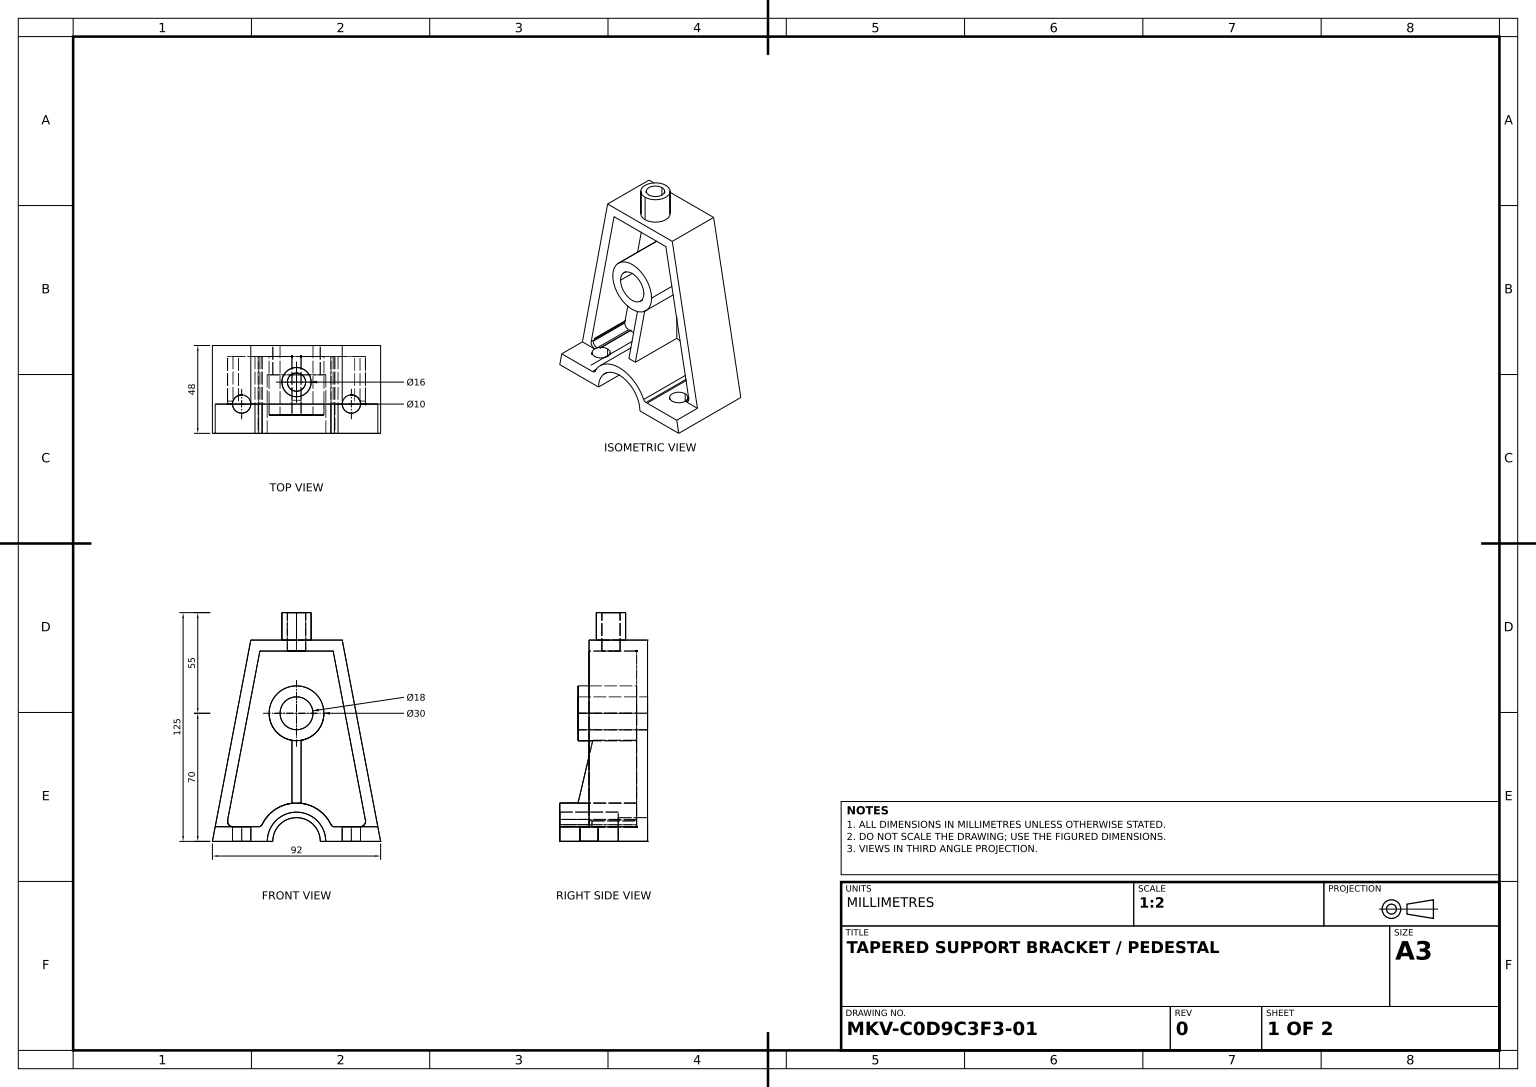
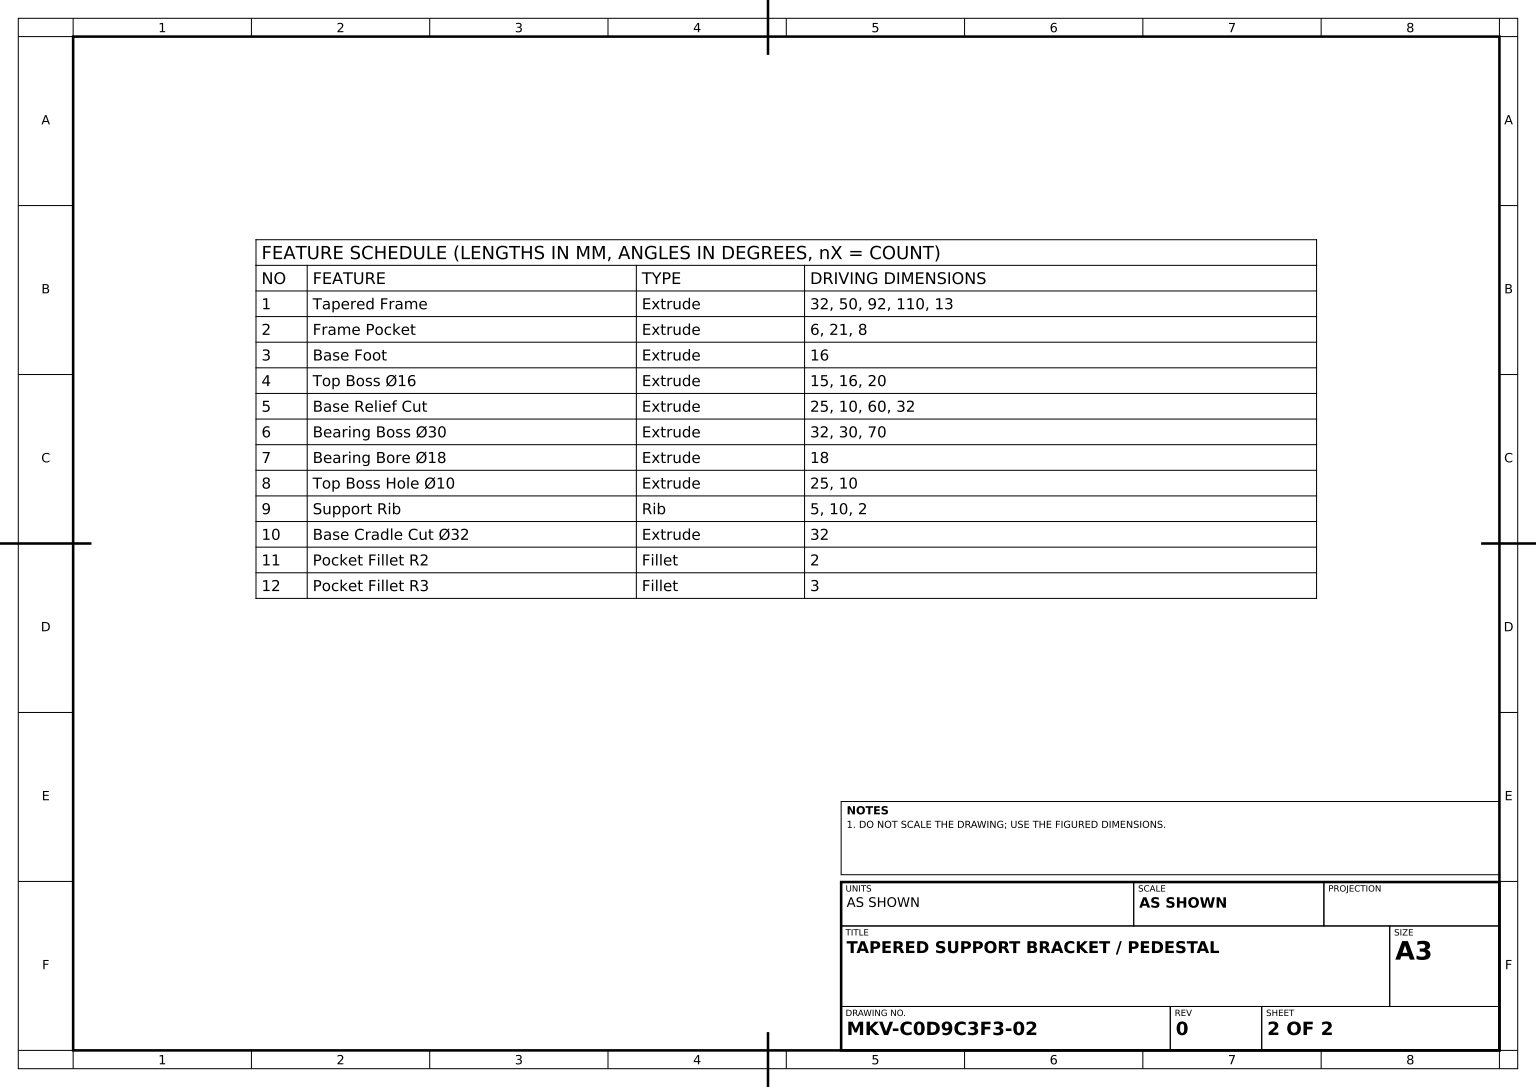
ISO-10303-21;
HEADER;
FILE_DESCRIPTION((''),'2;1');
FILE_NAME('','',(''),(''),'','','');
FILE_SCHEMA(('AUTOMOTIVE_DESIGN'));
ENDSEC;
DATA;
#1=APPLICATION_CONTEXT('');
#2=PRODUCT_CONTEXT('',#1,'mechanical');
#3=PRODUCT('','','',(#2));
#4=PRODUCT_DEFINITION_FORMATION('','',#3);
#5=PRODUCT_DEFINITION_CONTEXT('',#1,'design');
#6=PRODUCT_DEFINITION('','',#4,#5);
#7=PRODUCT_DEFINITION_SHAPE('','',#6);
#8=(LENGTH_UNIT()NAMED_UNIT(*)SI_UNIT(.MILLI.,.METRE.));
#9=(NAMED_UNIT(*)PLANE_ANGLE_UNIT()SI_UNIT($,.RADIAN.));
#10=(NAMED_UNIT(*)SI_UNIT($,.STERADIAN.)SOLID_ANGLE_UNIT());
#11=UNCERTAINTY_MEASURE_WITH_UNIT(LENGTH_MEASURE(1.E-05),#8,'distance_accuracy_value','');
#12=(GEOMETRIC_REPRESENTATION_CONTEXT(3)GLOBAL_UNCERTAINTY_ASSIGNED_CONTEXT((#11))GLOBAL_UNIT_ASSIGNED_CONTEXT((#8,#9,#10))REPRESENTATION_CONTEXT('',''));
#13=CARTESIAN_POINT('',(13.,0.,16.));
#14=VERTEX_POINT('',#13);
#15=CARTESIAN_POINT('',(13.,0.,0.));
#16=VERTEX_POINT('',#15);
#17=CARTESIAN_POINT('',(13.,0.,32.));
#18=DIRECTION('',(0.,0.,-1.));
#19=VECTOR('',#18,1000.);
#20=LINE('',#17,#19);
#21=EDGE_CURVE('',#14,#16,#20,.T.);
#22=ORIENTED_EDGE('',*,*,#21,.F.);
#23=CARTESIAN_POINT('',(-13.,0.,16.));
#24=VERTEX_POINT('',#23);
#25=CARTESIAN_POINT('',(0.,0.,16.));
#26=DIRECTION('',(1.,0.,0.));
#27=AXIS2_PLACEMENT_3D('',#25,#18,#26);
#28=CIRCLE('',#27,13.);
#29=EDGE_CURVE('',#24,#14,#28,.T.);
#30=ORIENTED_EDGE('',*,*,#29,.F.);
#31=CARTESIAN_POINT('',(-13.,0.,0.));
#32=VERTEX_POINT('',#31);
#33=CARTESIAN_POINT('',(-13.,0.,32.));
#34=LINE('',#33,#19);
#35=EDGE_CURVE('',#24,#32,#34,.T.);
#36=ORIENTED_EDGE('',*,*,#35,.T.);
#37=CARTESIAN_POINT('',(0.,0.,0.));
#38=DIRECTION('',(-1.,0.,0.));
#39=AXIS2_PLACEMENT_3D('',#37,#18,#38);
#40=CIRCLE('',#39,13.);
#41=EDGE_CURVE('',#32,#16,#40,.T.);
#42=ORIENTED_EDGE('',*,*,#41,.T.);
#43=EDGE_LOOP('',(#22,#30,#36,#42));
#44=FACE_OUTER_BOUND('',#43,.T.);
#45=CARTESIAN_POINT('',(0.,0.,32.));
#46=AXIS2_PLACEMENT_3D('',#45,#18,#38);
#47=CYLINDRICAL_SURFACE('',#46,13.);
#48=ADVANCED_FACE('',(#44),#47,.F.);
#49=CARTESIAN_POINT('',(44.472727,8.,48.));
#50=VERTEX_POINT('',#49);
#51=CARTESIAN_POINT('',(44.472727,8.,32.));
#52=VERTEX_POINT('',#51);
#53=LINE('',#49,#19);
#54=EDGE_CURVE('',#50,#52,#53,.T.);
#55=ORIENTED_EDGE('',*,*,#54,.T.);
#56=CARTESIAN_POINT('',(35.,8.,32.));
#57=VERTEX_POINT('',#56);
#58=CARTESIAN_POINT('',(0.,8.,32.));
#59=VECTOR('',#26,1000.);
#60=LINE('',#58,#59);
#61=EDGE_CURVE('',#57,#52,#60,.T.);
#62=ORIENTED_EDGE('',*,*,#61,.F.);
#63=CARTESIAN_POINT('',(30.,8.,37.));
#64=VERTEX_POINT('',#63);
#65=CARTESIAN_POINT('',(30.,8.,32.));
#66=DIRECTION('',(0.,1.,0.));
#67=DIRECTION('',(0.,0.,1.));
#68=AXIS2_PLACEMENT_3D('',#65,#66,#67);
#69=CIRCLE('',#68,5.);
#70=EDGE_CURVE('',#64,#57,#69,.T.);
#71=ORIENTED_EDGE('',*,*,#70,.F.);
#72=CARTESIAN_POINT('',(30.,8.,27.));
#73=VERTEX_POINT('',#72);
#74=EDGE_CURVE('',#73,#64,#69,.T.);
#75=ORIENTED_EDGE('',*,*,#74,.F.);
#76=CARTESIAN_POINT('',(34.737459,8.,30.401101));
#77=VERTEX_POINT('',#76);
#78=EDGE_CURVE('',#77,#73,#69,.T.);
#79=ORIENTED_EDGE('',*,*,#78,.F.);
#80=CARTESIAN_POINT('',(34.737459,8.,6.));
#81=VERTEX_POINT('',#80);
#82=LINE('',#80,#19);
#83=EDGE_CURVE('',#77,#81,#82,.T.);
#84=ORIENTED_EDGE('',*,*,#83,.T.);
#85=CARTESIAN_POINT('',(20.712315,8.,6.));
#86=VERTEX_POINT('',#85);
#87=CARTESIAN_POINT('',(19.416488,8.,6.));
#88=LINE('',#87,#59);
#89=EDGE_CURVE('',#86,#81,#88,.T.);
#90=ORIENTED_EDGE('',*,*,#89,.F.);
#91=CARTESIAN_POINT('',(20.712315,8.,48.));
#92=VERTEX_POINT('',#91);
#93=VECTOR('',#67,1000.);
#94=LINE('',#91,#93);
#95=EDGE_CURVE('',#86,#92,#94,.T.);
#96=ORIENTED_EDGE('',*,*,#95,.T.);
#97=CARTESIAN_POINT('',(0.,8.,48.));
#98=LINE('',#97,#59);
#99=EDGE_CURVE('',#92,#50,#98,.T.);
#100=ORIENTED_EDGE('',*,*,#99,.T.);
#101=EDGE_LOOP('',(#55,#62,#71,#75,#79,#84,#90,#96,#100));
#102=FACE_OUTER_BOUND('',#101,.T.);
#103=CARTESIAN_POINT('',(19.416488,8.,-122.895478));
#104=DIRECTION('',(0.,-1.,0.));
#105=AXIS2_PLACEMENT_3D('',#103,#104,#18);
#106=PLANE('',#105);
#107=ADVANCED_FACE('',(#102),#106,.F.);
#108=CARTESIAN_POINT('',(0.,125.,12.));
#109=VERTEX_POINT('',#108);
#110=CARTESIAN_POINT('',(0.,110.,12.));
#111=VERTEX_POINT('',#110);
#112=VECTOR('',#104,1000.);
#113=LINE('',#108,#112);
#114=EDGE_CURVE('',#109,#111,#113,.T.);
#115=ORIENTED_EDGE('',*,*,#114,.T.);
#116=CARTESIAN_POINT('',(0.,110.,28.));
#117=VERTEX_POINT('',#116);
#118=CARTESIAN_POINT('',(0.,110.,20.));
#119=AXIS2_PLACEMENT_3D('',#118,#66,#67);
#120=CIRCLE('',#119,8.);
#121=EDGE_CURVE('',#111,#117,#120,.T.);
#122=ORIENTED_EDGE('',*,*,#121,.T.);
#123=CARTESIAN_POINT('',(0.,125.,28.));
#124=VERTEX_POINT('',#123);
#125=LINE('',#123,#112);
#126=EDGE_CURVE('',#124,#117,#125,.T.);
#127=ORIENTED_EDGE('',*,*,#126,.F.);
#128=CARTESIAN_POINT('',(0.,125.,20.));
#129=AXIS2_PLACEMENT_3D('',#128,#66,#67);
#130=CIRCLE('',#129,8.);
#131=EDGE_CURVE('',#109,#124,#130,.T.);
#132=ORIENTED_EDGE('',*,*,#131,.F.);
#133=EDGE_LOOP('',(#115,#122,#127,#132));
#134=FACE_OUTER_BOUND('',#133,.T.);
#135=AXIS2_PLACEMENT_3D('',#128,#104,#18);
#136=CYLINDRICAL_SURFACE('',#135,8.);
#137=ADVANCED_FACE('',(#134),#136,.T.);
#138=CARTESIAN_POINT('',(-9.,70.,38.));
#139=VERTEX_POINT('',#138);
#140=CARTESIAN_POINT('',(9.,70.,38.));
#141=VERTEX_POINT('',#140);
#142=CARTESIAN_POINT('',(0.,70.,38.));
#143=AXIS2_PLACEMENT_3D('',#142,#67,#26);
#144=CIRCLE('',#143,9.);
#145=EDGE_CURVE('',#139,#141,#144,.T.);
#146=ORIENTED_EDGE('',*,*,#145,.F.);
#147=EDGE_CURVE('',#141,#139,#144,.T.);
#148=ORIENTED_EDGE('',*,*,#147,.F.);
#149=EDGE_LOOP('',(#146,#148));
#150=FACE_BOUND('',#149,.T.);
#151=CARTESIAN_POINT('',(15.,70.,38.));
#152=VERTEX_POINT('',#151);
#153=CARTESIAN_POINT('',(-15.,70.,38.));
#154=VERTEX_POINT('',#153);
#155=CIRCLE('',#143,15.);
#156=EDGE_CURVE('',#152,#154,#155,.T.);
#157=ORIENTED_EDGE('',*,*,#156,.T.);
#158=EDGE_CURVE('',#154,#152,#155,.T.);
#159=ORIENTED_EDGE('',*,*,#158,.T.);
#160=EDGE_LOOP('',(#157,#159));
#161=FACE_OUTER_BOUND('',#160,.T.);
#162=PLANE('',#143);
#163=ADVANCED_FACE('',(#150,#161),#162,.T.);
#164=CARTESIAN_POINT('',(-25.,110.,32.));
#165=VERTEX_POINT('',#164);
#166=CARTESIAN_POINT('',(-25.,110.,0.));
#167=VERTEX_POINT('',#166);
#168=LINE('',#164,#19);
#169=EDGE_CURVE('',#165,#167,#168,.T.);
#170=ORIENTED_EDGE('',*,*,#169,.F.);
#171=CARTESIAN_POINT('',(25.,110.,32.));
#172=VERTEX_POINT('',#171);
#173=VECTOR('',#38,1000.);
#174=LINE('',#171,#173);
#175=EDGE_CURVE('',#172,#165,#174,.T.);
#176=ORIENTED_EDGE('',*,*,#175,.F.);
#177=CARTESIAN_POINT('',(25.,110.,0.));
#178=VERTEX_POINT('',#177);
#179=LINE('',#171,#19);
#180=EDGE_CURVE('',#172,#178,#179,.T.);
#181=ORIENTED_EDGE('',*,*,#180,.T.);
#182=LINE('',#177,#173);
#183=EDGE_CURVE('',#178,#167,#182,.T.);
#184=ORIENTED_EDGE('',*,*,#183,.T.);
#185=EDGE_LOOP('',(#170,#176,#181,#184));
#186=FACE_OUTER_BOUND('',#185,.T.);
#187=EDGE_CURVE('',#117,#111,#120,.T.);
#188=ORIENTED_EDGE('',*,*,#187,.F.);
#189=ORIENTED_EDGE('',*,*,#121,.F.);
#190=EDGE_LOOP('',(#188,#189));
#191=FACE_BOUND('',#190,.T.);
#192=AXIS2_PLACEMENT_3D('',#171,#104,#18);
#193=PLANE('',#192);
#194=ADVANCED_FACE('',(#186,#191),#193,.F.);
#195=CARTESIAN_POINT('',(-46.,0.,48.));
#196=VERTEX_POINT('',#195);
#197=CARTESIAN_POINT('',(-46.,0.,0.));
#198=VERTEX_POINT('',#197);
#199=CARTESIAN_POINT('',(-46.,0.,32.));
#200=LINE('',#199,#19);
#201=EDGE_CURVE('',#196,#198,#200,.T.);
#202=ORIENTED_EDGE('',*,*,#201,.F.);
#203=CARTESIAN_POINT('',(-44.472727,8.,48.));
#204=VERTEX_POINT('',#203);
#205=CARTESIAN_POINT('',(-44.382426,8.473009,48.));
#206=DIRECTION('',(-0.187522425,-0.982260322,0.));
#207=VECTOR('',#206,1000.);
#208=LINE('',#205,#207);
#209=EDGE_CURVE('',#204,#196,#208,.T.);
#210=ORIENTED_EDGE('',*,*,#209,.F.);
#211=CARTESIAN_POINT('',(-44.472727,8.,32.));
#212=VERTEX_POINT('',#211);
#213=LINE('',#203,#19);
#214=EDGE_CURVE('',#204,#212,#213,.T.);
#215=ORIENTED_EDGE('',*,*,#214,.T.);
#216=LINE('',#164,#207);
#217=EDGE_CURVE('',#165,#212,#216,.T.);
#218=ORIENTED_EDGE('',*,*,#217,.F.);
#219=ORIENTED_EDGE('',*,*,#169,.T.);
#220=LINE('',#166,#207);
#221=EDGE_CURVE('',#167,#198,#220,.T.);
#222=ORIENTED_EDGE('',*,*,#221,.T.);
#223=EDGE_LOOP('',(#202,#210,#215,#218,#219,#222));
#224=FACE_OUTER_BOUND('',#223,.T.);
#225=DIRECTION('',(0.982260322,-0.187522425,0.));
#226=DIRECTION('',(0.187522425,0.982260322,0.));
#227=AXIS2_PLACEMENT_3D('',#164,#225,#226);
#228=PLANE('',#227);
#229=ADVANCED_FACE('',(#224),#228,.F.);
#230=CARTESIAN_POINT('',(0.,104.,15.));
#231=VERTEX_POINT('',#230);
#232=CARTESIAN_POINT('',(0.,104.,25.));
#233=VERTEX_POINT('',#232);
#234=CARTESIAN_POINT('',(0.,104.,20.));
#235=AXIS2_PLACEMENT_3D('',#234,#66,#67);
#236=CIRCLE('',#235,5.);
#237=EDGE_CURVE('',#231,#233,#236,.T.);
#238=ORIENTED_EDGE('',*,*,#237,.T.);
#239=EDGE_CURVE('',#233,#231,#236,.T.);
#240=ORIENTED_EDGE('',*,*,#239,.T.);
#241=EDGE_LOOP('',(#238,#240));
#242=FACE_BOUND('',#241,.T.);
#243=CARTESIAN_POINT('',(20.037094,104.,6.));
#244=VERTEX_POINT('',#243);
#245=CARTESIAN_POINT('',(20.037094,104.,32.));
#246=VERTEX_POINT('',#245);
#247=CARTESIAN_POINT('',(20.037094,104.,-122.895478));
#248=LINE('',#247,#93);
#249=EDGE_CURVE('',#244,#246,#248,.T.);
#250=ORIENTED_EDGE('',*,*,#249,.T.);
#251=CARTESIAN_POINT('',(-20.037094,104.,32.));
#252=VERTEX_POINT('',#251);
#253=LINE('',#245,#173);
#254=EDGE_CURVE('',#246,#252,#253,.T.);
#255=ORIENTED_EDGE('',*,*,#254,.T.);
#256=CARTESIAN_POINT('',(-20.037094,104.,6.));
#257=VERTEX_POINT('',#256);
#258=CARTESIAN_POINT('',(-20.037094,104.,-122.895478));
#259=LINE('',#258,#93);
#260=EDGE_CURVE('',#257,#252,#259,.T.);
#261=ORIENTED_EDGE('',*,*,#260,.F.);
#262=LINE('',#243,#173);
#263=EDGE_CURVE('',#244,#257,#262,.T.);
#264=ORIENTED_EDGE('',*,*,#263,.F.);
#265=EDGE_LOOP('',(#250,#255,#261,#264));
#266=FACE_OUTER_BOUND('',#265,.T.);
#267=AXIS2_PLACEMENT_3D('',#247,#66,#67);
#268=PLANE('',#267);
#269=ADVANCED_FACE('',(#242,#266),#268,.F.);
#270=CARTESIAN_POINT('',(2.5,20.850659,6.));
#271=VERTEX_POINT('',#270);
#272=CARTESIAN_POINT('',(18.911244,9.130435,6.));
#273=VERTEX_POINT('',#272);
#274=CARTESIAN_POINT('',(0.,0.,6.));
#275=AXIS2_PLACEMENT_3D('',#274,#18,#38);
#276=CIRCLE('',#275,21.);
#277=EDGE_CURVE('',#271,#273,#276,.T.);
#278=ORIENTED_EDGE('',*,*,#277,.T.);
#279=CARTESIAN_POINT('',(20.712315,10.,6.));
#280=AXIS2_PLACEMENT_3D('',#279,#67,#38);
#281=CIRCLE('',#280,2.);
#282=EDGE_CURVE('',#273,#86,#281,.T.);
#283=ORIENTED_EDGE('',*,*,#282,.T.);
#284=ORIENTED_EDGE('',*,*,#89,.T.);
#285=CARTESIAN_POINT('',(37.68424,11.562567,6.));
#286=VERTEX_POINT('',#285);
#287=CARTESIAN_POINT('',(34.737459,11.,6.));
#288=AXIS2_PLACEMENT_3D('',#287,#67,#38);
#289=CIRCLE('',#288,3.);
#290=EDGE_CURVE('',#81,#286,#289,.T.);
#291=ORIENTED_EDGE('',*,*,#290,.T.);
#292=CARTESIAN_POINT('',(38.364367,8.,6.));
#293=DIRECTION('',(-0.187522425,0.982260322,0.));
#294=VECTOR('',#293,1000.);
#295=LINE('',#292,#294);
#296=EDGE_CURVE('',#286,#244,#295,.T.);
#297=ORIENTED_EDGE('',*,*,#296,.T.);
#298=ORIENTED_EDGE('',*,*,#263,.T.);
#299=CARTESIAN_POINT('',(-37.68424,11.562567,6.));
#300=VERTEX_POINT('',#299);
#301=LINE('',#256,#207);
#302=EDGE_CURVE('',#257,#300,#301,.T.);
#303=ORIENTED_EDGE('',*,*,#302,.T.);
#304=CARTESIAN_POINT('',(-37.737459,11.,6.));
#305=VERTEX_POINT('',#304);
#306=CARTESIAN_POINT('',(-34.737459,11.,6.));
#307=AXIS2_PLACEMENT_3D('',#306,#67,#38);
#308=CIRCLE('',#307,3.);
#309=EDGE_CURVE('',#300,#305,#308,.T.);
#310=ORIENTED_EDGE('',*,*,#309,.T.);
#311=CARTESIAN_POINT('',(-34.737459,8.,6.));
#312=VERTEX_POINT('',#311);
#313=EDGE_CURVE('',#305,#312,#308,.T.);
#314=ORIENTED_EDGE('',*,*,#313,.T.);
#315=CARTESIAN_POINT('',(-20.712315,8.,6.));
#316=VERTEX_POINT('',#315);
#317=CARTESIAN_POINT('',(-38.364367,8.,6.));
#318=LINE('',#317,#59);
#319=EDGE_CURVE('',#312,#316,#318,.T.);
#320=ORIENTED_EDGE('',*,*,#319,.T.);
#321=CARTESIAN_POINT('',(-18.911244,9.130435,6.));
#322=VERTEX_POINT('',#321);
#323=CARTESIAN_POINT('',(-20.712315,10.,6.));
#324=AXIS2_PLACEMENT_3D('',#323,#67,#38);
#325=CIRCLE('',#324,2.);
#326=EDGE_CURVE('',#316,#322,#325,.T.);
#327=ORIENTED_EDGE('',*,*,#326,.T.);
#328=CARTESIAN_POINT('',(-2.5,20.850659,6.));
#329=VERTEX_POINT('',#328);
#330=EDGE_CURVE('',#322,#329,#276,.T.);
#331=ORIENTED_EDGE('',*,*,#330,.T.);
#332=CARTESIAN_POINT('',(-2.5,55.209801,6.));
#333=VERTEX_POINT('',#332);
#334=CARTESIAN_POINT('',(-2.5,0.,6.));
#335=LINE('',#334,#112);
#336=EDGE_CURVE('',#333,#329,#335,.T.);
#337=ORIENTED_EDGE('',*,*,#336,.F.);
#338=CARTESIAN_POINT('',(-15.,70.,6.));
#339=VERTEX_POINT('',#338);
#340=CARTESIAN_POINT('',(0.,70.,6.));
#341=AXIS2_PLACEMENT_3D('',#340,#67,#38);
#342=CIRCLE('',#341,15.);
#343=EDGE_CURVE('',#339,#333,#342,.T.);
#344=ORIENTED_EDGE('',*,*,#343,.F.);
#345=CARTESIAN_POINT('',(15.,70.,6.));
#346=VERTEX_POINT('',#345);
#347=EDGE_CURVE('',#346,#339,#342,.T.);
#348=ORIENTED_EDGE('',*,*,#347,.F.);
#349=CARTESIAN_POINT('',(2.5,55.209801,6.));
#350=VERTEX_POINT('',#349);
#351=EDGE_CURVE('',#350,#346,#342,.T.);
#352=ORIENTED_EDGE('',*,*,#351,.F.);
#353=CARTESIAN_POINT('',(2.5,0.,6.));
#354=LINE('',#353,#112);
#355=EDGE_CURVE('',#350,#271,#354,.T.);
#356=ORIENTED_EDGE('',*,*,#355,.T.);
#357=EDGE_LOOP('',(#278,#283,#284,#291,#297,#298,#303,#310,#314,#320,#327,#331,#337,#344,#348,#352,#356));
#358=FACE_OUTER_BOUND('',#357,.T.);
#359=PLANE('',#275);
#360=ADVANCED_FACE('',(#358),#359,.F.);
#361=ORIENTED_EDGE('',*,*,#126,.T.);
#362=ORIENTED_EDGE('',*,*,#187,.T.);
#363=ORIENTED_EDGE('',*,*,#114,.F.);
#364=EDGE_CURVE('',#124,#109,#130,.T.);
#365=ORIENTED_EDGE('',*,*,#364,.F.);
#366=EDGE_LOOP('',(#361,#362,#363,#365));
#367=FACE_OUTER_BOUND('',#366,.T.);
#368=ADVANCED_FACE('',(#367),#136,.T.);
#369=ORIENTED_EDGE('',*,*,#70,.T.);
#370=EDGE_CURVE('',#57,#77,#69,.T.);
#371=ORIENTED_EDGE('',*,*,#370,.T.);
#372=ORIENTED_EDGE('',*,*,#78,.T.);
#373=CARTESIAN_POINT('',(30.,0.,27.));
#374=VERTEX_POINT('',#373);
#375=CARTESIAN_POINT('',(30.,-17.,27.));
#376=VECTOR('',#66,1000.);
#377=LINE('',#375,#376);
#378=EDGE_CURVE('',#374,#73,#377,.T.);
#379=ORIENTED_EDGE('',*,*,#378,.F.);
#380=CARTESIAN_POINT('',(30.,0.,37.));
#381=VERTEX_POINT('',#380);
#382=CARTESIAN_POINT('',(30.,0.,32.));
#383=AXIS2_PLACEMENT_3D('',#382,#66,#67);
#384=CIRCLE('',#383,5.);
#385=EDGE_CURVE('',#381,#374,#384,.T.);
#386=ORIENTED_EDGE('',*,*,#385,.F.);
#387=CARTESIAN_POINT('',(30.,-17.,37.));
#388=LINE('',#387,#376);
#389=EDGE_CURVE('',#381,#64,#388,.T.);
#390=ORIENTED_EDGE('',*,*,#389,.T.);
#391=EDGE_LOOP('',(#369,#371,#372,#379,#386,#390));
#392=FACE_OUTER_BOUND('',#391,.T.);
#393=CARTESIAN_POINT('',(30.,-17.,32.));
#394=AXIS2_PLACEMENT_3D('',#393,#66,#67);
#395=CYLINDRICAL_SURFACE('',#394,5.);
#396=ADVANCED_FACE('',(#392),#395,.F.);
#397=CARTESIAN_POINT('',(-18.911244,9.130435,48.));
#398=VERTEX_POINT('',#397);
#399=CARTESIAN_POINT('',(-20.712315,8.,48.));
#400=VERTEX_POINT('',#399);
#401=CARTESIAN_POINT('',(-20.712315,10.,48.));
#402=AXIS2_PLACEMENT_3D('',#401,#18,#26);
#403=CIRCLE('',#402,2.);
#404=EDGE_CURVE('',#398,#400,#403,.T.);
#405=ORIENTED_EDGE('',*,*,#404,.F.);
#406=CARTESIAN_POINT('',(-18.911244,9.130435,-122.895478));
#407=LINE('',#406,#93);
#408=EDGE_CURVE('',#322,#398,#407,.T.);
#409=ORIENTED_EDGE('',*,*,#408,.F.);
#410=ORIENTED_EDGE('',*,*,#326,.F.);
#411=LINE('',#315,#19);
#412=EDGE_CURVE('',#400,#316,#411,.T.);
#413=ORIENTED_EDGE('',*,*,#412,.F.);
#414=EDGE_LOOP('',(#405,#409,#410,#413));
#415=FACE_OUTER_BOUND('',#414,.T.);
#416=CARTESIAN_POINT('',(-20.712315,10.,-122.895478));
#417=AXIS2_PLACEMENT_3D('',#416,#67,#26);
#418=CYLINDRICAL_SURFACE('',#417,2.);
#419=ADVANCED_FACE('',(#415),#418,.F.);
#420=CARTESIAN_POINT('',(-2.5,55.209801,29.950635));
#421=VERTEX_POINT('',#420);
#422=CARTESIAN_POINT('',(2.5,55.209801,29.950635));
#423=VERTEX_POINT('',#422);
#424=CARTESIAN_POINT('',(-0.841177,54.929408,30.01661));
#425=CARTESIAN_POINT('',(0.841177,54.929408,30.01661));
#426=(BOUNDED_CURVE()B_SPLINE_CURVE(3,(#420,#424,#425,#422),.UNSPECIFIED.,.F.,.T.)B_SPLINE_CURVE_WITH_KNOTS((4,4),(2.974144574,3.309040733),.UNSPECIFIED.)CURVE()GEOMETRIC_REPRESENTATION_ITEM()RATIONAL_B_SPLINE_CURVE((1.,0.990675531,0.990675531,1.))REPRESENTATION_ITEM(''));
#427=EDGE_CURVE('',#421,#423,#426,.T.);
#428=ORIENTED_EDGE('',*,*,#427,.F.);
#429=CARTESIAN_POINT('',(-2.5,20.850659,38.035139));
#430=VERTEX_POINT('',#429);
#431=CARTESIAN_POINT('',(-2.5,55.,30.));
#432=DIRECTION('',(0.,-0.973417168,0.229039334));
#433=VECTOR('',#432,1000.);
#434=LINE('',#431,#433);
#435=EDGE_CURVE('',#421,#430,#434,.T.);
#436=ORIENTED_EDGE('',*,*,#435,.T.);
#437=CARTESIAN_POINT('',(2.5,20.850659,38.035139));
#438=VERTEX_POINT('',#437);
#439=CARTESIAN_POINT('',(0.837303,21.050017,37.988231));
#440=CARTESIAN_POINT('',(-0.837303,21.050017,37.988231));
#441=(BOUNDED_CURVE()B_SPLINE_CURVE(3,(#437,#439,#440,#429),.UNSPECIFIED.,.F.,.T.)B_SPLINE_CURVE_WITH_KNOTS((4,4),(3.022262029,3.260923278),.UNSPECIFIED.)CURVE()GEOMETRIC_REPRESENTATION_ITEM()RATIONAL_B_SPLINE_CURVE((1.,0.995259031,0.995259031,1.))REPRESENTATION_ITEM(''));
#442=EDGE_CURVE('',#438,#430,#441,.T.);
#443=ORIENTED_EDGE('',*,*,#442,.F.);
#444=CARTESIAN_POINT('',(2.5,55.,30.));
#445=LINE('',#444,#433);
#446=EDGE_CURVE('',#423,#438,#445,.T.);
#447=ORIENTED_EDGE('',*,*,#446,.F.);
#448=EDGE_LOOP('',(#428,#436,#443,#447));
#449=FACE_OUTER_BOUND('',#448,.T.);
#450=CARTESIAN_POINT('',(0.,55.,30.));
#451=DIRECTION('',(0.,0.229039334,0.973417168));
#452=AXIS2_PLACEMENT_3D('',#450,#451,#432);
#453=PLANE('',#452);
#454=ADVANCED_FACE('',(#449),#453,.T.);
#455=CARTESIAN_POINT('',(18.911244,9.130435,48.));
#456=VERTEX_POINT('',#455);
#457=CARTESIAN_POINT('',(0.,0.,48.));
#458=AXIS2_PLACEMENT_3D('',#457,#67,#26);
#459=CIRCLE('',#458,21.);
#460=EDGE_CURVE('',#456,#398,#459,.T.);
#461=ORIENTED_EDGE('',*,*,#460,.F.);
#462=CARTESIAN_POINT('',(18.911244,9.130435,-122.895478));
#463=LINE('',#462,#19);
#464=EDGE_CURVE('',#456,#273,#463,.T.);
#465=ORIENTED_EDGE('',*,*,#464,.T.);
#466=ORIENTED_EDGE('',*,*,#277,.F.);
#467=CARTESIAN_POINT('',(2.5,20.850659,-122.895478));
#468=LINE('',#467,#93);
#469=EDGE_CURVE('',#271,#438,#468,.T.);
#470=ORIENTED_EDGE('',*,*,#469,.T.);
#471=ORIENTED_EDGE('',*,*,#442,.T.);
#472=CARTESIAN_POINT('',(-2.5,20.850659,-122.895478));
#473=LINE('',#472,#93);
#474=EDGE_CURVE('',#329,#430,#473,.T.);
#475=ORIENTED_EDGE('',*,*,#474,.F.);
#476=ORIENTED_EDGE('',*,*,#330,.F.);
#477=ORIENTED_EDGE('',*,*,#408,.T.);
#478=EDGE_LOOP('',(#461,#465,#466,#470,#471,#475,#476,#477));
#479=FACE_OUTER_BOUND('',#478,.T.);
#480=CARTESIAN_POINT('',(0.,0.,-122.895478));
#481=AXIS2_PLACEMENT_3D('',#480,#67,#26);
#482=CYLINDRICAL_SURFACE('',#481,21.);
#483=ADVANCED_FACE('',(#479),#482,.T.);
#484=ORIENTED_EDGE('',*,*,#427,.T.);
#485=CARTESIAN_POINT('',(2.5,55.209801,38.));
#486=LINE('',#485,#19);
#487=EDGE_CURVE('',#423,#350,#486,.T.);
#488=ORIENTED_EDGE('',*,*,#487,.T.);
#489=ORIENTED_EDGE('',*,*,#351,.T.);
#490=LINE('',#151,#19);
#491=EDGE_CURVE('',#152,#346,#490,.T.);
#492=ORIENTED_EDGE('',*,*,#491,.F.);
#493=ORIENTED_EDGE('',*,*,#158,.F.);
#494=LINE('',#153,#19);
#495=EDGE_CURVE('',#154,#339,#494,.T.);
#496=ORIENTED_EDGE('',*,*,#495,.T.);
#497=ORIENTED_EDGE('',*,*,#343,.T.);
#498=CARTESIAN_POINT('',(-2.5,55.209801,38.));
#499=LINE('',#498,#19);
#500=EDGE_CURVE('',#421,#333,#499,.T.);
#501=ORIENTED_EDGE('',*,*,#500,.F.);
#502=EDGE_LOOP('',(#484,#488,#489,#492,#493,#496,#497,#501));
#503=FACE_OUTER_BOUND('',#502,.T.);
#504=AXIS2_PLACEMENT_3D('',#142,#18,#38);
#505=CYLINDRICAL_SURFACE('',#504,15.);
#506=ADVANCED_FACE('',(#503),#505,.T.);
#507=CARTESIAN_POINT('',(-35.,8.,32.));
#508=VERTEX_POINT('',#507);
#509=CARTESIAN_POINT('',(-37.686402,11.551246,32.));
#510=VERTEX_POINT('',#509);
#511=CARTESIAN_POINT('',(-34.739621,10.988679,32.));
#512=AXIS2_PLACEMENT_3D('',#511,#18,#38);
#513=CIRCLE('',#512,3.);
#514=EDGE_CURVE('',#508,#510,#513,.T.);
#515=ORIENTED_EDGE('',*,*,#514,.F.);
#516=CARTESIAN_POINT('',(-34.737459,8.,30.401101));
#517=VERTEX_POINT('',#516);
#518=CARTESIAN_POINT('',(-30.,8.,32.));
#519=AXIS2_PLACEMENT_3D('',#518,#66,#67);
#520=CIRCLE('',#519,5.);
#521=EDGE_CURVE('',#517,#508,#520,.T.);
#522=ORIENTED_EDGE('',*,*,#521,.F.);
#523=CARTESIAN_POINT('',(-37.737459,11.,30.401101));
#524=VERTEX_POINT('',#523);
#525=CARTESIAN_POINT('',(-34.737459,11.,30.401101));
#526=AXIS2_PLACEMENT_3D('',#525,#67,#104);
#527=CIRCLE('',#526,3.);
#528=EDGE_CURVE('',#524,#517,#527,.T.);
#529=ORIENTED_EDGE('',*,*,#528,.F.);
#530=CARTESIAN_POINT('',(-37.68424,11.562567,30.401101));
#531=VERTEX_POINT('',#530);
#532=EDGE_CURVE('',#531,#524,#527,.T.);
#533=ORIENTED_EDGE('',*,*,#532,.F.);
#534=CARTESIAN_POINT('',(-37.686402,11.551246,31.467006));
#535=CARTESIAN_POINT('',(-37.68424,11.562567,30.934095));
#536=B_SPLINE_CURVE_WITH_KNOTS('',3,(#509,#534,#535,#530),.UNSPECIFIED.,.F.,.F.,(4,4),(0.,0.00159894),.UNSPECIFIED.);
#537=EDGE_CURVE('',#510,#531,#536,.T.);
#538=ORIENTED_EDGE('',*,*,#537,.F.);
#539=EDGE_LOOP('',(#515,#522,#529,#533,#538));
#540=FACE_OUTER_BOUND('',#539,.T.);
#541=CARTESIAN_POINT('',(-38.309325,8.288315,32.));
#542=CARTESIAN_POINT('',(-37.686402,11.551246,31.733506));
#543=CARTESIAN_POINT('',(-38.309325,8.288315,31.717244));
#544=CARTESIAN_POINT('',(-35.,8.,31.718801));
#545=CARTESIAN_POINT('',(-37.685987,11.55342,31.467025));
#546=CARTESIAN_POINT('',(-38.313874,8.264487,31.432093));
#547=CARTESIAN_POINT('',(-34.975824,8.,31.437887));
#548=CARTESIAN_POINT('',(-37.684901,11.559107,30.934069));
#549=CARTESIAN_POINT('',(-38.332064,8.169204,30.890538));
#550=CARTESIAN_POINT('',(-34.884831,8.,30.898536));
#551=CARTESIAN_POINT('',(-37.68424,11.562567,30.667594));
#552=CARTESIAN_POINT('',(-38.346023,8.096088,30.630402));
#553=CARTESIAN_POINT('',(-34.818166,8.,30.640232));
#554=CARTESIAN_POINT('',(-38.364367,8.,30.401101));
#555=(BOUNDED_SURFACE()B_SPLINE_SURFACE(3,2,((#509,#541,#507),(#542,#543,#544),(#545,#546,#547),(#548,#549,#550),(#551,#552,#553),(#530,#554,#516)),.UNSPECIFIED.,.F.,.F.,.F.)B_SPLINE_SURFACE_WITH_KNOTS((4,2,4),(3,3),(0.005636624,0.006435659,0.007234694),(0.,1.),.UNSPECIFIED.)GEOMETRIC_REPRESENTATION_ITEM()RATIONAL_B_SPLINE_SURFACE(((1.,0.670238249,1.),(1.,0.670252841,1.),(1.,0.667302878,1.),(1.,0.656046208,1.),(1.,0.647746586,1.),(1.,0.637368643,1.)))REPRESENTATION_ITEM('')SURFACE());
#556=ADVANCED_FACE('',(#540),#555,.F.);
#557=ORIENTED_EDGE('',*,*,#29,.T.);
#558=CARTESIAN_POINT('',(16.,0.,16.));
#559=VERTEX_POINT('',#558);
#560=LINE('',#13,#59);
#561=EDGE_CURVE('',#14,#559,#560,.T.);
#562=ORIENTED_EDGE('',*,*,#561,.T.);
#563=CARTESIAN_POINT('',(-16.,0.,16.));
#564=VERTEX_POINT('',#563);
#565=AXIS2_PLACEMENT_3D('',#25,#67,#26);
#566=CIRCLE('',#565,16.);
#567=EDGE_CURVE('',#559,#564,#566,.T.);
#568=ORIENTED_EDGE('',*,*,#567,.T.);
#569=CARTESIAN_POINT('',(-46.,0.,16.));
#570=LINE('',#569,#59);
#571=EDGE_CURVE('',#564,#24,#570,.T.);
#572=ORIENTED_EDGE('',*,*,#571,.T.);
#573=EDGE_LOOP('',(#557,#562,#568,#572));
#574=FACE_OUTER_BOUND('',#573,.T.);
#575=PLANE('',#565);
#576=ADVANCED_FACE('',(#574),#575,.T.);
#577=CARTESIAN_POINT('',(-16.,0.,48.));
#578=VERTEX_POINT('',#577);
#579=LINE('',#457,#59);
#580=EDGE_CURVE('',#196,#578,#579,.T.);
#581=ORIENTED_EDGE('',*,*,#580,.F.);
#582=ORIENTED_EDGE('',*,*,#201,.T.);
#583=LINE('',#197,#59);
#584=EDGE_CURVE('',#198,#32,#583,.T.);
#585=ORIENTED_EDGE('',*,*,#584,.T.);
#586=ORIENTED_EDGE('',*,*,#35,.F.);
#587=ORIENTED_EDGE('',*,*,#571,.F.);
#588=LINE('',#563,#93);
#589=EDGE_CURVE('',#564,#578,#588,.T.);
#590=ORIENTED_EDGE('',*,*,#589,.T.);
#591=EDGE_LOOP('',(#581,#582,#585,#586,#587,#590));
#592=FACE_OUTER_BOUND('',#591,.T.);
#593=CARTESIAN_POINT('',(-30.,0.,27.));
#594=VERTEX_POINT('',#593);
#595=CARTESIAN_POINT('',(-30.,0.,37.));
#596=VERTEX_POINT('',#595);
#597=CARTESIAN_POINT('',(-30.,0.,32.));
#598=AXIS2_PLACEMENT_3D('',#597,#66,#67);
#599=CIRCLE('',#598,5.);
#600=EDGE_CURVE('',#594,#596,#599,.T.);
#601=ORIENTED_EDGE('',*,*,#600,.T.);
#602=EDGE_CURVE('',#596,#594,#599,.T.);
#603=ORIENTED_EDGE('',*,*,#602,.T.);
#604=EDGE_LOOP('',(#601,#603));
#605=FACE_BOUND('',#604,.T.);
#606=AXIS2_PLACEMENT_3D('',#199,#66,#67);
#607=PLANE('',#606);
#608=ADVANCED_FACE('',(#592,#605),#607,.F.);
#609=ORIENTED_EDGE('',*,*,#446,.T.);
#610=ORIENTED_EDGE('',*,*,#469,.F.);
#611=ORIENTED_EDGE('',*,*,#355,.F.);
#612=ORIENTED_EDGE('',*,*,#487,.F.);
#613=EDGE_LOOP('',(#609,#610,#611,#612));
#614=FACE_OUTER_BOUND('',#613,.T.);
#615=CARTESIAN_POINT('',(2.5,62.5,24.));
#616=AXIS2_PLACEMENT_3D('',#615,#26,#18);
#617=PLANE('',#616);
#618=ADVANCED_FACE('',(#614),#617,.T.);
#619=CARTESIAN_POINT('',(0.,125.,15.));
#620=VERTEX_POINT('',#619);
#621=CARTESIAN_POINT('',(0.,100.,15.));
#622=LINE('',#621,#376);
#623=EDGE_CURVE('',#231,#620,#622,.T.);
#624=ORIENTED_EDGE('',*,*,#623,.F.);
#625=ORIENTED_EDGE('',*,*,#239,.F.);
#626=CARTESIAN_POINT('',(0.,125.,25.));
#627=VERTEX_POINT('',#626);
#628=CARTESIAN_POINT('',(0.,100.,25.));
#629=LINE('',#628,#376);
#630=EDGE_CURVE('',#233,#627,#629,.T.);
#631=ORIENTED_EDGE('',*,*,#630,.T.);
#632=CIRCLE('',#129,5.);
#633=EDGE_CURVE('',#627,#620,#632,.T.);
#634=ORIENTED_EDGE('',*,*,#633,.T.);
#635=EDGE_LOOP('',(#624,#625,#631,#634));
#636=FACE_OUTER_BOUND('',#635,.T.);
#637=CARTESIAN_POINT('',(0.,100.,20.));
#638=AXIS2_PLACEMENT_3D('',#637,#66,#67);
#639=CYLINDRICAL_SURFACE('',#638,5.);
#640=ADVANCED_FACE('',(#636),#639,.F.);
#641=LINE('',#299,#19);
#642=EDGE_CURVE('',#531,#300,#641,.T.);
#643=ORIENTED_EDGE('',*,*,#642,.T.);
#644=ORIENTED_EDGE('',*,*,#302,.F.);
#645=ORIENTED_EDGE('',*,*,#260,.T.);
#646=LINE('',#251,#207);
#647=EDGE_CURVE('',#252,#510,#646,.T.);
#648=ORIENTED_EDGE('',*,*,#647,.T.);
#649=ORIENTED_EDGE('',*,*,#537,.T.);
#650=EDGE_LOOP('',(#643,#644,#645,#648,#649));
#651=FACE_OUTER_BOUND('',#650,.T.);
#652=DIRECTION('',(-0.982260322,0.187522425,0.));
#653=AXIS2_PLACEMENT_3D('',#258,#652,#206);
#654=PLANE('',#653);
#655=ADVANCED_FACE('',(#651),#654,.F.);
#656=ORIENTED_EDGE('',*,*,#54,.F.);
#657=CARTESIAN_POINT('',(46.,0.,48.));
#658=VERTEX_POINT('',#657);
#659=CARTESIAN_POINT('',(44.382426,8.473009,48.));
#660=LINE('',#659,#294);
#661=EDGE_CURVE('',#658,#50,#660,.T.);
#662=ORIENTED_EDGE('',*,*,#661,.F.);
#663=CARTESIAN_POINT('',(46.,0.,0.));
#664=VERTEX_POINT('',#663);
#665=CARTESIAN_POINT('',(46.,0.,32.));
#666=LINE('',#665,#19);
#667=EDGE_CURVE('',#658,#664,#666,.T.);
#668=ORIENTED_EDGE('',*,*,#667,.T.);
#669=LINE('',#663,#294);
#670=EDGE_CURVE('',#664,#178,#669,.T.);
#671=ORIENTED_EDGE('',*,*,#670,.T.);
#672=ORIENTED_EDGE('',*,*,#180,.F.);
#673=LINE('',#665,#294);
#674=EDGE_CURVE('',#52,#172,#673,.T.);
#675=ORIENTED_EDGE('',*,*,#674,.F.);
#676=EDGE_LOOP('',(#656,#662,#668,#671,#672,#675));
#677=FACE_OUTER_BOUND('',#676,.T.);
#678=DIRECTION('',(-0.982260322,-0.187522425,0.));
#679=DIRECTION('',(0.187522425,-0.982260322,0.));
#680=AXIS2_PLACEMENT_3D('',#665,#678,#679);
#681=PLANE('',#680);
#682=ADVANCED_FACE('',(#677),#681,.F.);
#683=CARTESIAN_POINT('',(9.,70.,0.));
#684=VERTEX_POINT('',#683);
#685=LINE('',#683,#93);
#686=EDGE_CURVE('',#684,#141,#685,.T.);
#687=ORIENTED_EDGE('',*,*,#686,.F.);
#688=CARTESIAN_POINT('',(-9.,70.,0.));
#689=VERTEX_POINT('',#688);
#690=CARTESIAN_POINT('',(0.,70.,0.));
#691=AXIS2_PLACEMENT_3D('',#690,#67,#26);
#692=CIRCLE('',#691,9.);
#693=EDGE_CURVE('',#689,#684,#692,.T.);
#694=ORIENTED_EDGE('',*,*,#693,.F.);
#695=LINE('',#688,#93);
#696=EDGE_CURVE('',#689,#139,#695,.T.);
#697=ORIENTED_EDGE('',*,*,#696,.T.);
#698=ORIENTED_EDGE('',*,*,#145,.T.);
#699=EDGE_LOOP('',(#687,#694,#697,#698));
#700=FACE_OUTER_BOUND('',#699,.T.);
#701=CYLINDRICAL_SURFACE('',#691,9.);
#702=ADVANCED_FACE('',(#700),#701,.F.);
#703=ORIENTED_EDGE('',*,*,#435,.F.);
#704=ORIENTED_EDGE('',*,*,#500,.T.);
#705=ORIENTED_EDGE('',*,*,#336,.T.);
#706=ORIENTED_EDGE('',*,*,#474,.T.);
#707=EDGE_LOOP('',(#703,#704,#705,#706));
#708=FACE_OUTER_BOUND('',#707,.T.);
#709=CARTESIAN_POINT('',(-2.5,62.5,24.));
#710=AXIS2_PLACEMENT_3D('',#709,#26,#18);
#711=PLANE('',#710);
#712=ADVANCED_FACE('',(#708),#711,.F.);
#713=EDGE_CURVE('',#684,#689,#692,.T.);
#714=ORIENTED_EDGE('',*,*,#713,.F.);
#715=ORIENTED_EDGE('',*,*,#686,.T.);
#716=ORIENTED_EDGE('',*,*,#147,.T.);
#717=ORIENTED_EDGE('',*,*,#696,.F.);
#718=EDGE_LOOP('',(#714,#715,#716,#717));
#719=FACE_OUTER_BOUND('',#718,.T.);
#720=ADVANCED_FACE('',(#719),#701,.F.);
#721=CARTESIAN_POINT('',(37.686402,11.551246,32.));
#722=VERTEX_POINT('',#721);
#723=CARTESIAN_POINT('',(38.364367,8.,32.));
#724=LINE('',#723,#294);
#725=EDGE_CURVE('',#722,#246,#724,.T.);
#726=ORIENTED_EDGE('',*,*,#725,.F.);
#727=CARTESIAN_POINT('',(34.739621,10.988679,32.));
#728=AXIS2_PLACEMENT_3D('',#727,#18,#38);
#729=CIRCLE('',#728,3.);
#730=EDGE_CURVE('',#722,#57,#729,.T.);
#731=ORIENTED_EDGE('',*,*,#730,.T.);
#732=ORIENTED_EDGE('',*,*,#61,.T.);
#733=ORIENTED_EDGE('',*,*,#674,.T.);
#734=ORIENTED_EDGE('',*,*,#175,.T.);
#735=ORIENTED_EDGE('',*,*,#217,.T.);
#736=LINE('',#58,#173);
#737=EDGE_CURVE('',#508,#212,#736,.T.);
#738=ORIENTED_EDGE('',*,*,#737,.F.);
#739=ORIENTED_EDGE('',*,*,#514,.T.);
#740=ORIENTED_EDGE('',*,*,#647,.F.);
#741=ORIENTED_EDGE('',*,*,#254,.F.);
#742=EDGE_LOOP('',(#726,#731,#732,#733,#734,#735,#738,#739,#740,#741));
#743=FACE_OUTER_BOUND('',#742,.T.);
#744=PLANE('',#46);
#745=ADVANCED_FACE('',(#743),#744,.F.);
#746=ORIENTED_EDGE('',*,*,#725,.T.);
#747=ORIENTED_EDGE('',*,*,#249,.F.);
#748=ORIENTED_EDGE('',*,*,#296,.F.);
#749=CARTESIAN_POINT('',(37.68424,11.562567,30.401101));
#750=VERTEX_POINT('',#749);
#751=CARTESIAN_POINT('',(37.68424,11.562567,32.));
#752=LINE('',#751,#93);
#753=EDGE_CURVE('',#286,#750,#752,.T.);
#754=ORIENTED_EDGE('',*,*,#753,.T.);
#755=CARTESIAN_POINT('',(37.68424,11.562567,30.934095));
#756=CARTESIAN_POINT('',(37.686402,11.551246,31.467006));
#757=B_SPLINE_CURVE_WITH_KNOTS('',3,(#749,#755,#756,#721),.UNSPECIFIED.,.F.,.F.,(4,4),(0.,0.00159894),.UNSPECIFIED.);
#758=EDGE_CURVE('',#750,#722,#757,.T.);
#759=ORIENTED_EDGE('',*,*,#758,.T.);
#760=EDGE_LOOP('',(#746,#747,#748,#754,#759));
#761=FACE_OUTER_BOUND('',#760,.T.);
#762=CARTESIAN_POINT('',(38.364367,8.,-122.895478));
#763=DIRECTION('',(0.982260322,0.187522425,0.));
#764=AXIS2_PLACEMENT_3D('',#762,#763,#293);
#765=PLANE('',#764);
#766=ADVANCED_FACE('',(#761),#765,.F.);
#767=ORIENTED_EDGE('',*,*,#370,.F.);
#768=ORIENTED_EDGE('',*,*,#730,.F.);
#769=ORIENTED_EDGE('',*,*,#758,.F.);
#770=CARTESIAN_POINT('',(34.737459,11.,30.401101));
#771=AXIS2_PLACEMENT_3D('',#770,#67,#26);
#772=CIRCLE('',#771,3.);
#773=EDGE_CURVE('',#77,#750,#772,.T.);
#774=ORIENTED_EDGE('',*,*,#773,.F.);
#775=EDGE_LOOP('',(#767,#768,#769,#774));
#776=FACE_OUTER_BOUND('',#775,.T.);
#777=CARTESIAN_POINT('',(38.309325,8.288315,32.));
#778=CARTESIAN_POINT('',(35.,8.,31.718801));
#779=CARTESIAN_POINT('',(38.309325,8.288315,31.717244));
#780=CARTESIAN_POINT('',(37.686402,11.551246,31.733506));
#781=CARTESIAN_POINT('',(34.975824,8.,31.437887));
#782=CARTESIAN_POINT('',(38.313874,8.264487,31.432093));
#783=CARTESIAN_POINT('',(37.685987,11.55342,31.467025));
#784=CARTESIAN_POINT('',(34.884831,8.,30.898536));
#785=CARTESIAN_POINT('',(38.332064,8.169204,30.890538));
#786=CARTESIAN_POINT('',(37.684901,11.559107,30.934069));
#787=CARTESIAN_POINT('',(34.818166,8.,30.640232));
#788=CARTESIAN_POINT('',(38.346023,8.096088,30.630402));
#789=CARTESIAN_POINT('',(37.68424,11.562567,30.667594));
#790=CARTESIAN_POINT('',(38.364367,8.,30.401101));
#791=(BOUNDED_SURFACE()B_SPLINE_SURFACE(3,2,((#56,#777,#721),(#778,#779,#780),(#781,#782,#783),(#784,#785,#786),(#787,#788,#789),(#76,#790,#749)),.UNSPECIFIED.,.F.,.F.,.F.)B_SPLINE_SURFACE_WITH_KNOTS((4,2,4),(3,3),(0.005636624,0.006435659,0.007234694),(0.,1.),.UNSPECIFIED.)GEOMETRIC_REPRESENTATION_ITEM()RATIONAL_B_SPLINE_SURFACE(((1.,0.670238249,1.),(1.,0.670252841,1.),(1.,0.667302878,1.),(1.,0.656046208,1.),(1.,0.647746586,1.),(1.,0.637368643,1.)))REPRESENTATION_ITEM('')SURFACE());
#792=ADVANCED_FACE('',(#776),#791,.F.);
#793=CARTESIAN_POINT('',(-30.,8.,37.));
#794=VERTEX_POINT('',#793);
#795=CARTESIAN_POINT('',(-30.,8.,27.));
#796=VERTEX_POINT('',#795);
#797=EDGE_CURVE('',#794,#796,#520,.T.);
#798=ORIENTED_EDGE('',*,*,#797,.T.);
#799=CARTESIAN_POINT('',(-30.,-17.,27.));
#800=LINE('',#799,#376);
#801=EDGE_CURVE('',#594,#796,#800,.T.);
#802=ORIENTED_EDGE('',*,*,#801,.F.);
#803=ORIENTED_EDGE('',*,*,#602,.F.);
#804=CARTESIAN_POINT('',(-30.,-17.,37.));
#805=LINE('',#804,#376);
#806=EDGE_CURVE('',#596,#794,#805,.T.);
#807=ORIENTED_EDGE('',*,*,#806,.T.);
#808=EDGE_LOOP('',(#798,#802,#803,#807));
#809=FACE_OUTER_BOUND('',#808,.T.);
#810=CARTESIAN_POINT('',(-30.,-17.,32.));
#811=AXIS2_PLACEMENT_3D('',#810,#66,#67);
#812=CYLINDRICAL_SURFACE('',#811,5.);
#813=ADVANCED_FACE('',(#809),#812,.F.);
#814=ORIENTED_EDGE('',*,*,#661,.T.);
#815=ORIENTED_EDGE('',*,*,#99,.F.);
#816=CARTESIAN_POINT('',(20.712315,10.,48.));
#817=AXIS2_PLACEMENT_3D('',#816,#18,#26);
#818=CIRCLE('',#817,2.);
#819=EDGE_CURVE('',#92,#456,#818,.T.);
#820=ORIENTED_EDGE('',*,*,#819,.T.);
#821=ORIENTED_EDGE('',*,*,#460,.T.);
#822=ORIENTED_EDGE('',*,*,#404,.T.);
#823=LINE('',#97,#173);
#824=EDGE_CURVE('',#400,#204,#823,.T.);
#825=ORIENTED_EDGE('',*,*,#824,.T.);
#826=ORIENTED_EDGE('',*,*,#209,.T.);
#827=ORIENTED_EDGE('',*,*,#580,.T.);
#828=CARTESIAN_POINT('',(16.,0.,48.));
#829=VERTEX_POINT('',#828);
#830=CIRCLE('',#458,16.);
#831=EDGE_CURVE('',#829,#578,#830,.T.);
#832=ORIENTED_EDGE('',*,*,#831,.F.);
#833=EDGE_CURVE('',#829,#658,#579,.T.);
#834=ORIENTED_EDGE('',*,*,#833,.T.);
#835=EDGE_LOOP('',(#814,#815,#820,#821,#822,#825,#826,#827,#832,#834));
#836=FACE_OUTER_BOUND('',#835,.T.);
#837=PLANE('',#458);
#838=ADVANCED_FACE('',(#836),#837,.T.);
#839=ORIENTED_EDGE('',*,*,#833,.F.);
#840=LINE('',#558,#19);
#841=EDGE_CURVE('',#829,#559,#840,.T.);
#842=ORIENTED_EDGE('',*,*,#841,.T.);
#843=ORIENTED_EDGE('',*,*,#561,.F.);
#844=ORIENTED_EDGE('',*,*,#21,.T.);
#845=LINE('',#15,#59);
#846=EDGE_CURVE('',#16,#664,#845,.T.);
#847=ORIENTED_EDGE('',*,*,#846,.T.);
#848=ORIENTED_EDGE('',*,*,#667,.F.);
#849=EDGE_LOOP('',(#839,#842,#843,#844,#847,#848));
#850=FACE_OUTER_BOUND('',#849,.T.);
#851=EDGE_CURVE('',#374,#381,#384,.T.);
#852=ORIENTED_EDGE('',*,*,#851,.T.);
#853=ORIENTED_EDGE('',*,*,#385,.T.);
#854=EDGE_LOOP('',(#852,#853));
#855=FACE_BOUND('',#854,.T.);
#856=AXIS2_PLACEMENT_3D('',#17,#66,#67);
#857=PLANE('',#856);
#858=ADVANCED_FACE('',(#850,#855),#857,.F.);
#859=CARTESIAN_POINT('',(-34.737459,8.,32.));
#860=LINE('',#859,#93);
#861=EDGE_CURVE('',#312,#517,#860,.T.);
#862=ORIENTED_EDGE('',*,*,#861,.T.);
#863=EDGE_CURVE('',#796,#517,#520,.T.);
#864=ORIENTED_EDGE('',*,*,#863,.F.);
#865=ORIENTED_EDGE('',*,*,#797,.F.);
#866=EDGE_CURVE('',#508,#794,#520,.T.);
#867=ORIENTED_EDGE('',*,*,#866,.F.);
#868=ORIENTED_EDGE('',*,*,#737,.T.);
#869=ORIENTED_EDGE('',*,*,#214,.F.);
#870=ORIENTED_EDGE('',*,*,#824,.F.);
#871=ORIENTED_EDGE('',*,*,#412,.T.);
#872=ORIENTED_EDGE('',*,*,#319,.F.);
#873=EDGE_LOOP('',(#862,#864,#865,#867,#868,#869,#870,#871,#872));
#874=FACE_OUTER_BOUND('',#873,.T.);
#875=CARTESIAN_POINT('',(-38.364367,8.,-122.895478));
#876=AXIS2_PLACEMENT_3D('',#875,#104,#26);
#877=PLANE('',#876);
#878=ADVANCED_FACE('',(#874),#877,.F.);
#879=EDGE_CURVE('',#620,#627,#632,.T.);
#880=ORIENTED_EDGE('',*,*,#879,.F.);
#881=ORIENTED_EDGE('',*,*,#633,.F.);
#882=EDGE_LOOP('',(#880,#881));
#883=FACE_BOUND('',#882,.T.);
#884=ORIENTED_EDGE('',*,*,#364,.T.);
#885=ORIENTED_EDGE('',*,*,#131,.T.);
#886=EDGE_LOOP('',(#884,#885));
#887=FACE_OUTER_BOUND('',#886,.T.);
#888=PLANE('',#129);
#889=ADVANCED_FACE('',(#883,#887),#888,.T.);
#890=ORIENTED_EDGE('',*,*,#347,.T.);
#891=ORIENTED_EDGE('',*,*,#495,.F.);
#892=ORIENTED_EDGE('',*,*,#156,.F.);
#893=ORIENTED_EDGE('',*,*,#491,.T.);
#894=EDGE_LOOP('',(#890,#891,#892,#893));
#895=FACE_OUTER_BOUND('',#894,.T.);
#896=ADVANCED_FACE('',(#895),#505,.T.);
#897=ORIENTED_EDGE('',*,*,#528,.T.);
#898=ORIENTED_EDGE('',*,*,#861,.F.);
#899=ORIENTED_EDGE('',*,*,#313,.F.);
#900=CARTESIAN_POINT('',(-37.737459,11.,-122.895478));
#901=LINE('',#900,#19);
#902=EDGE_CURVE('',#524,#305,#901,.T.);
#903=ORIENTED_EDGE('',*,*,#902,.F.);
#904=EDGE_LOOP('',(#897,#898,#899,#903));
#905=FACE_OUTER_BOUND('',#904,.T.);
#906=CARTESIAN_POINT('',(-34.737459,11.,-122.895478));
#907=AXIS2_PLACEMENT_3D('',#906,#18,#38);
#908=CYLINDRICAL_SURFACE('',#907,3.);
#909=ADVANCED_FACE('',(#905),#908,.F.);
#910=ORIENTED_EDGE('',*,*,#841,.F.);
#911=ORIENTED_EDGE('',*,*,#831,.T.);
#912=ORIENTED_EDGE('',*,*,#589,.F.);
#913=ORIENTED_EDGE('',*,*,#567,.F.);
#914=EDGE_LOOP('',(#910,#911,#912,#913));
#915=FACE_OUTER_BOUND('',#914,.T.);
#916=CYLINDRICAL_SURFACE('',#565,16.);
#917=ADVANCED_FACE('',(#915),#916,.F.);
#918=ORIENTED_EDGE('',*,*,#773,.T.);
#919=ORIENTED_EDGE('',*,*,#753,.F.);
#920=ORIENTED_EDGE('',*,*,#290,.F.);
#921=ORIENTED_EDGE('',*,*,#83,.F.);
#922=EDGE_LOOP('',(#918,#919,#920,#921));
#923=FACE_OUTER_BOUND('',#922,.T.);
#924=CARTESIAN_POINT('',(34.737459,11.,-122.895478));
#925=AXIS2_PLACEMENT_3D('',#924,#18,#38);
#926=CYLINDRICAL_SURFACE('',#925,3.);
#927=ADVANCED_FACE('',(#923),#926,.F.);
#928=ORIENTED_EDGE('',*,*,#389,.F.);
#929=ORIENTED_EDGE('',*,*,#851,.F.);
#930=ORIENTED_EDGE('',*,*,#378,.T.);
#931=ORIENTED_EDGE('',*,*,#74,.T.);
#932=EDGE_LOOP('',(#928,#929,#930,#931));
#933=FACE_OUTER_BOUND('',#932,.T.);
#934=ADVANCED_FACE('',(#933),#395,.F.);
#935=ORIENTED_EDGE('',*,*,#670,.F.);
#936=ORIENTED_EDGE('',*,*,#846,.F.);
#937=ORIENTED_EDGE('',*,*,#41,.F.);
#938=ORIENTED_EDGE('',*,*,#584,.F.);
#939=ORIENTED_EDGE('',*,*,#221,.F.);
#940=ORIENTED_EDGE('',*,*,#183,.F.);
#941=EDGE_LOOP('',(#935,#936,#937,#938,#939,#940));
#942=FACE_OUTER_BOUND('',#941,.T.);
#943=ORIENTED_EDGE('',*,*,#693,.T.);
#944=ORIENTED_EDGE('',*,*,#713,.T.);
#945=EDGE_LOOP('',(#943,#944));
#946=FACE_BOUND('',#945,.T.);
#947=PLANE('',#39);
#948=ADVANCED_FACE('',(#942,#946),#947,.T.);
#949=ORIENTED_EDGE('',*,*,#630,.F.);
#950=ORIENTED_EDGE('',*,*,#237,.F.);
#951=ORIENTED_EDGE('',*,*,#623,.T.);
#952=ORIENTED_EDGE('',*,*,#879,.T.);
#953=EDGE_LOOP('',(#949,#950,#951,#952));
#954=FACE_OUTER_BOUND('',#953,.T.);
#955=ADVANCED_FACE('',(#954),#639,.F.);
#956=ORIENTED_EDGE('',*,*,#600,.F.);
#957=ORIENTED_EDGE('',*,*,#801,.T.);
#958=ORIENTED_EDGE('',*,*,#863,.T.);
#959=ORIENTED_EDGE('',*,*,#521,.T.);
#960=ORIENTED_EDGE('',*,*,#866,.T.);
#961=ORIENTED_EDGE('',*,*,#806,.F.);
#962=EDGE_LOOP('',(#956,#957,#958,#959,#960,#961));
#963=FACE_OUTER_BOUND('',#962,.T.);
#964=ADVANCED_FACE('',(#963),#812,.F.);
#965=ORIENTED_EDGE('',*,*,#532,.T.);
#966=ORIENTED_EDGE('',*,*,#902,.T.);
#967=ORIENTED_EDGE('',*,*,#309,.F.);
#968=ORIENTED_EDGE('',*,*,#642,.F.);
#969=EDGE_LOOP('',(#965,#966,#967,#968));
#970=FACE_OUTER_BOUND('',#969,.T.);
#971=ADVANCED_FACE('',(#970),#908,.F.);
#972=ORIENTED_EDGE('',*,*,#282,.F.);
#973=ORIENTED_EDGE('',*,*,#464,.F.);
#974=ORIENTED_EDGE('',*,*,#819,.F.);
#975=ORIENTED_EDGE('',*,*,#95,.F.);
#976=EDGE_LOOP('',(#972,#973,#974,#975));
#977=FACE_OUTER_BOUND('',#976,.T.);
#978=CARTESIAN_POINT('',(20.712315,10.,-122.895478));
#979=AXIS2_PLACEMENT_3D('',#978,#67,#26);
#980=CYLINDRICAL_SURFACE('',#979,2.);
#981=ADVANCED_FACE('',(#977),#980,.F.);
#982=CLOSED_SHELL('',(#48,#107,#137,#163,#194,#229,#269,#360,#368,#396,#419,#454,#483,#506,#556,#576,#608,#618,#640,#655,#682,#702,#712,#720,#745,#766,#792,#813,#838,#858,#878,#889,#896,#909,#917,#927,#934,#948,#955,#964,#971,#981));
#983=MANIFOLD_SOLID_BREP('',#982);
#984=ADVANCED_BREP_SHAPE_REPRESENTATION('',(#983),#12);
#985=SHAPE_DEFINITION_REPRESENTATION(#7,#984);
ENDSEC;
END-ISO-10303-21;
